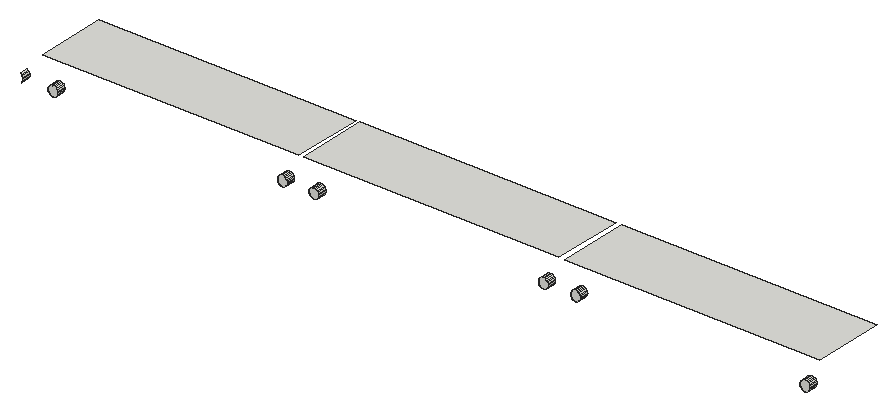
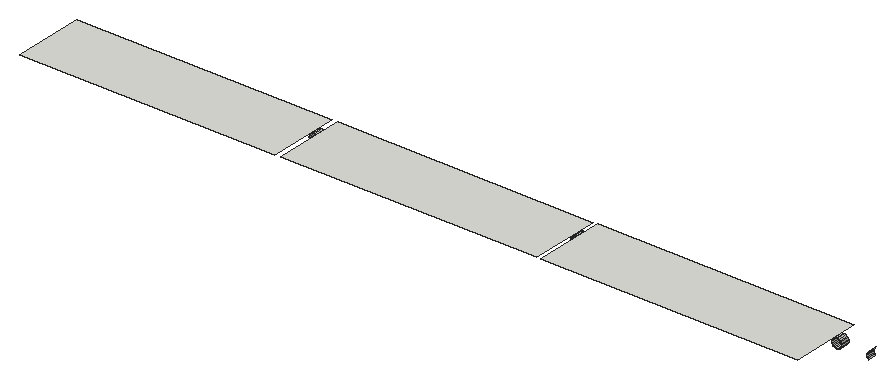
# SketchUp Ruby script. Lengths in inches.
U = 1.inch
M = Sketchup.active_model
def pt(a) = Geom::Point3d.new(a.map { |v| v * U })
def face(e, loops, mat)
  f = e.add_face(loops[0].map { |a| pt(a) })
  loops[1..].each { |l| e.add_face(l.map { |a| pt(a) }).erase! }
  f.material = f.back_material = mat if mat
  f
end
# faces: each face lists its corners as indices into pts; further lists are holes
def faces(e, pts, list, mat = nil) = list.each { |f| face(e, (f[0].is_a?(Array) ? f : [f]).map { |l| l.map { |i| pts[i] } }, mat) }
# xy, xz, yz: faces in a plane at the given z, y or x. An outline is a flat list of corners, or four numbers for a rectangle; further outlines are holes
def ring(l) = l.size == 4 ? [[l[0], l[1]], [l[2], l[1]], [l[2], l[3]], [l[0], l[3]]] : l.each_slice(2).to_a
def flat(e, list, mat, &to3) = list.each { |f| face(e, (f[0].is_a?(Array) ? f : [f]).map { |l| ring(l).map { |u, v| to3.(u, v) } }, mat) }
def xy(e, z, list, mat = nil) = flat(e, list, mat) { |x, y| [x, y, z] }
def xz(e, y, list, mat = nil) = flat(e, list, mat) { |x, z| [x, y, z] }
def yz(e, x, list, mat = nil) = flat(e, list, mat) { |y, z| [x, y, z] }
def lines(e, pts, list) = list.each { |a, b| e.add_line(pt(pts[a]), pt(pts[b])) }
# prism: a flat outline (further loops are holes) pulled along v
def prism(e, loops, v, mat = nil)
  f = face(e, loops, mat); d = Geom::Vector3d.new(v.map { |x| x * U })
  f.pushpull(f.normal.samedirection?(d) ? d.length : -d.length)
end
def box(e, o, s, mat = nil) = prism(e, [[o, [o[0] + s[0], o[1], o[2]], [o[0] + s[0], o[1] + s[1], o[2]], [o[0], o[1] + s[1], o[2]]]], [0, 0, s[2]], mat)
def at(x, y, z, deg = 0) = Geom::Transformation.translation(pt([x, y, z])) * Geom::Transformation.rotation(ORIGIN, Z_AXIS, deg.degrees)
def axes(o, x, y, z) = Geom::Transformation.new([*x, 0, *y, 0, *z, 0, *pt(o).to_a, 1])
def part(name) = M.definitions.add(name)
# library, detail: a bought-in or finely detailed component or shape, given as its bounding box
def library(name, o, s) = part(name).tap { |d| box(d.entities, o, s) }
def detail(e, o, s) = box(e.add_group.entities, o, s)
def put(e, d, t, mat = nil) = e.add_instance(d, t).tap { |i| i.material = mat if mat }
def group(e, t, mat = nil) = e.add_group.tap { |g| g.transformation = t; g.material = mat if mat }.entities
root = M.entities
xy(root,138.0625,[[907.71,801.78,964.82,817.6],[965.89,801.78,1022.875,817.6],[1024.1875,801.78,1080.92,817.6]])
xz(root,799.91,[[911.6,131.88,911.89,131.92,912.16,132.03,912.39,132.21,912.57,132.44,912.68,132.71,912.72,133,912.68,133.29,912.57,133.57,912.39,133.8,912.16,133.98,911.89,134.09,911.6,134.13,911.3,134.09,911.03,133.98,910.8,133.8,910.62,133.57,910.51,133.29,910.47,133,910.51,132.71,910.62,132.44,910.8,132.21,911.03,132.03,911.3,131.92],[962.72,131.88,963.01,131.92,963.28,132.03,963.52,132.21,963.7,132.44,963.81,132.71,963.85,133,963.81,133.29,963.7,133.57,963.52,133.8,963.28,133.98,963.01,134.09,962.72,134.13,962.43,134.09,962.16,133.98,961.93,133.8,961.75,133.57,961.63,133.29,961.6,133,961.63,132.71,961.75,132.44,961.93,132.21,962.16,132.03,962.43,131.92],[969.77,131.88,970.0625,131.92,970.33,132.03,970.57,132.21,970.75,132.44,970.86,132.71,970.9,133,970.86,133.29,970.75,133.57,970.57,133.8,970.33,133.98,970.0625,134.09,969.77,134.13,969.48,134.09,969.21,133.98,968.98,133.8,968.8,133.57,968.69,133.29,968.65,133,968.69,132.71,968.8,132.44,968.98,132.21,969.21,132.03,969.48,131.92],[1020.9,131.88,1021.1875,131.92,1021.46,132.03,1021.69,132.21,1021.87,132.44,1021.98,132.71,1022.02,133,1021.98,133.29,1021.87,133.57,1021.69,133.8,1021.46,133.98,1021.1875,134.09,1020.9,134.13,1020.61,134.09,1020.33,133.98,1020.1,133.8,1019.92,133.57,1019.81,133.29,1019.77,133,1019.81,132.71,1019.92,132.44,1020.1,132.21,1020.33,132.03,1020.61,131.92],[1028.07,131.88,1028.36,131.92,1028.64,132.03,1028.87,132.21,1029.05,132.44,1029.16,132.71,1029.2,133,1029.16,133.29,1029.05,133.57,1028.87,133.8,1028.64,133.98,1028.36,134.09,1028.07,134.13,1027.78,134.09,1027.51,133.98,1027.28,133.8,1027.1,133.57,1026.99,133.29,1026.95,133,1026.99,132.71,1027.1,132.44,1027.28,132.21,1027.51,132.03,1027.78,131.92],
  [1079.2,131.88,1079.49,131.92,1079.76,132.03,1079.99,132.21,1080.17,132.44,1080.28,132.71,1080.32,133,1080.28,133.29,1080.17,133.57,1079.99,133.8,1079.76,133.98,1079.49,134.09,1079.2,134.13,1078.91,134.09,1078.64,133.98,1078.4,133.8,1078.22,133.57,1078.11,133.29,1078.07,133,1078.11,132.71,1078.22,132.44,1078.4,132.21,1078.64,132.03,1078.91,131.92]])
p = [[911.03,801.78,132.03],[911.3,801.78,131.92],[911.3,799.91,131.92],[911.03,799.91,132.03],[911.6,801.78,131.88],[911.6,799.91,131.88],
  [911.89,801.78,131.92],[911.89,799.91,131.92],[912.16,801.78,132.03],[912.16,799.91,132.03],[962.16,801.78,132.03],[962.43,801.78,131.92],
  [962.43,799.91,131.92],[962.16,799.91,132.03],[962.72,801.78,131.88],[962.72,799.91,131.88],[963.01,801.78,131.92],[963.01,799.91,131.92],
  [963.28,801.78,132.03],[963.28,799.91,132.03],[969.21,801.78,132.03],[969.48,801.78,131.92],[969.48,799.91,131.92],[969.21,799.91,132.03],
  [969.77,801.78,131.88],[969.77,799.91,131.88],[970.0625,801.78,131.92],[970.0625,799.91,131.92],[970.33,801.78,132.03],[970.33,799.91,132.03],
  [1020.33,801.78,132.03],[1020.61,801.78,131.92],[1020.61,799.91,131.92],[1020.33,799.91,132.03],[1020.9,801.78,131.88],[1020.9,799.91,131.88],
  [1021.1875,801.78,131.92],[1021.1875,799.91,131.92],[1021.46,801.78,132.03],[1021.46,799.91,132.03],[1027.51,801.78,132.03],[1027.78,801.78,131.92],
  [1027.78,799.91,131.92],[1027.51,799.91,132.03],[1028.07,801.78,131.88],[1028.07,799.91,131.88],[1028.36,801.78,131.92],[1028.36,799.91,131.92],
  [1028.64,801.78,132.03],[1028.64,799.91,132.03],[1078.64,801.78,132.03],[1078.91,801.78,131.92],[1078.91,799.91,131.92],[1078.64,799.91,132.03],
  [1079.2,801.78,131.88],[1079.2,799.91,131.88],[1079.49,801.78,131.92],[1079.49,799.91,131.92],[1079.76,801.78,132.03],[1079.76,799.91,132.03],
  [910.8,801.78,132.21],[910.8,799.91,132.21],[912.39,801.78,132.21],[912.39,799.91,132.21],[961.93,801.78,132.21],[961.93,799.91,132.21],
  [963.52,801.78,132.21],[963.52,799.91,132.21],[968.98,801.78,132.21],[968.98,799.91,132.21],[970.57,801.78,132.21],[970.57,799.91,132.21],
  [1020.1,801.78,132.21],[1020.1,799.91,132.21],[1021.69,801.78,132.21],[1021.69,799.91,132.21],[1027.28,801.78,132.21],[1027.28,799.91,132.21],
  [1028.87,801.78,132.21],[1028.87,799.91,132.21],[1078.4,801.78,132.21],[1078.4,799.91,132.21],[1079.99,801.78,132.21],[1079.99,799.91,132.21],
  [904.53,801.78,132.21],[904.71,801.78,132.44],[904.71,799.91,132.44],[904.53,799.91,132.21],[910.62,801.78,132.44],[910.62,799.91,132.44],
  [912.57,801.78,132.44],[912.57,799.91,132.44],[961.75,801.78,132.44],[961.75,799.91,132.44],[963.7,801.78,132.44],[963.7,799.91,132.44],
  [968.8,801.78,132.44],[968.8,799.91,132.44],[970.75,801.78,132.44],[970.75,799.91,132.44],[1019.92,801.78,132.44],[1019.92,799.91,132.44],
  [1021.87,801.78,132.44],[1021.87,799.91,132.44],[1027.1,801.78,132.44],[1027.1,799.91,132.44],[1029.05,801.78,132.44],[1029.05,799.91,132.44],
  [1078.22,801.78,132.44],[1078.22,799.91,132.44],[1080.17,801.78,132.44],[1080.17,799.91,132.44],[904.82,801.78,132.71],[904.82,799.91,132.71],
  [910.51,801.78,132.71],[910.51,799.91,132.71],[912.68,801.78,132.71],[912.68,799.91,132.71],[961.63,801.78,132.71],[961.63,799.91,132.71],
  [963.81,801.78,132.71],[963.81,799.91,132.71],[968.69,801.78,132.71],[968.69,799.91,132.71],[970.86,801.78,132.71],[970.86,799.91,132.71],
  [1019.81,801.78,132.71],[1019.81,799.91,132.71],[1021.98,801.78,132.71],[1021.98,799.91,132.71],[1026.99,801.78,132.71],[1026.99,799.91,132.71],
  [1029.16,801.78,132.71],[1029.16,799.91,132.71],[1078.11,801.78,132.71],[1078.11,799.91,132.71],[1080.28,801.78,132.71],[1080.28,799.91,132.71],
  [904.86,801.78,133],[904.86,799.91,133],[910.47,801.78,133],[910.47,799.91,133],[912.72,801.78,133],[912.72,799.91,133],
  [961.6,801.78,133],[961.6,799.91,133],[963.85,801.78,133],[963.85,799.91,133],[968.65,801.78,133],[968.65,799.91,133],
  [970.9,801.78,133],[970.9,799.91,133],[1019.77,801.78,133],[1019.77,799.91,133],[1022.02,801.78,133],[1022.02,799.91,133],
  [1026.95,801.78,133],[1026.95,799.91,133],[1029.2,801.78,133],[1029.2,799.91,133],[1078.07,801.78,133],[1078.07,799.91,133],
  [1080.32,801.78,133],[1080.32,799.91,133],[904.82,801.78,133.29],[904.82,799.91,133.29],[910.51,801.78,133.29],[910.51,799.91,133.29],
  [912.68,801.78,133.29],[912.68,799.91,133.29],[961.63,801.78,133.29],[961.63,799.91,133.29],[963.81,801.78,133.29],[963.81,799.91,133.29],
  [968.69,801.78,133.29],[968.69,799.91,133.29],[970.86,801.78,133.29],[970.86,799.91,133.29],[1019.81,801.78,133.29],[1019.81,799.91,133.29],
  [1021.98,801.78,133.29],[1021.98,799.91,133.29],[1026.99,801.78,133.29],[1026.99,799.91,133.29],[1029.16,801.78,133.29],[1029.16,799.91,133.29],
  [1078.11,801.78,133.29],[1078.11,799.91,133.29],[1080.28,801.78,133.29],[1080.28,799.91,133.29],[904.71,801.78,133.57],[904.71,799.91,133.57],
  [910.62,801.78,133.57],[910.62,799.91,133.57],[912.57,801.78,133.57],[912.57,799.91,133.57],[961.75,801.78,133.57],[961.75,799.91,133.57],
  [963.7,801.78,133.57],[963.7,799.91,133.57],[968.8,801.78,133.57],[968.8,799.91,133.57],[970.75,801.78,133.57],[970.75,799.91,133.57],
  [1019.92,801.78,133.57],[1019.92,799.91,133.57],[1021.87,801.78,133.57],[1021.87,799.91,133.57],[1027.1,801.78,133.57],[1027.1,799.91,133.57],
  [1029.05,801.78,133.57],[1029.05,799.91,133.57],[1078.22,801.78,133.57],[1078.22,799.91,133.57],[1080.17,801.78,133.57],[1080.17,799.91,133.57],
  [904.53,801.78,133.8],[904.53,799.91,133.8],[910.8,801.78,133.8],[910.8,799.91,133.8],[912.39,801.78,133.8],[912.39,799.91,133.8],
  [961.93,801.78,133.8],[961.93,799.91,133.8],[963.52,801.78,133.8],[963.52,799.91,133.8],[968.98,801.78,133.8],[968.98,799.91,133.8],
  [970.57,801.78,133.8],[970.57,799.91,133.8],[1020.1,801.78,133.8],[1020.1,799.91,133.8],[1021.69,801.78,133.8],[1021.69,799.91,133.8],
  [1027.28,801.78,133.8],[1027.28,799.91,133.8],[1028.87,801.78,133.8],[1028.87,799.91,133.8],[1078.4,801.78,133.8],[1078.4,799.91,133.8],
  [1079.99,801.78,133.8],[1079.99,799.91,133.8],[904.3,801.78,133.98],[904.3,799.91,133.98],[911.03,801.78,133.98],[911.03,799.91,133.98],
  [912.16,801.78,133.98],[912.16,799.91,133.98],[962.16,801.78,133.98],[962.16,799.91,133.98],[963.28,801.78,133.98],[963.28,799.91,133.98],
  [969.21,801.78,133.98],[969.21,799.91,133.98],[970.33,801.78,133.98],[970.33,799.91,133.98],[1020.33,801.78,133.98],[1020.33,799.91,133.98],
  [1021.46,801.78,133.98],[1021.46,799.91,133.98],[1027.51,801.78,133.98],[1027.51,799.91,133.98],[1028.64,801.78,133.98],[1028.64,799.91,133.98],
  [1078.64,801.78,133.98],[1078.64,799.91,133.98],[1079.76,801.78,133.98],[1079.76,799.91,133.98],[911.3,801.78,134.09],[911.3,799.91,134.09],
  [911.89,801.78,134.09],[911.89,799.91,134.09],[962.43,801.78,134.09],[962.43,799.91,134.09],[963.01,801.78,134.09],[963.01,799.91,134.09],
  [969.48,801.78,134.09],[969.48,799.91,134.09],[970.0625,801.78,134.09],[970.0625,799.91,134.09],[1020.61,801.78,134.09],[1020.61,799.91,134.09],
  [1021.1875,801.78,134.09],[1021.1875,799.91,134.09],[1027.78,801.78,134.09],[1027.78,799.91,134.09],[1028.36,801.78,134.09],[1028.36,799.91,134.09],
  [1078.91,801.78,134.09],[1078.91,799.91,134.09],[1079.49,801.78,134.09],[1079.49,799.91,134.09],[911.6,801.78,134.13],[911.6,799.91,134.13],
  [962.72,801.78,134.13],[962.72,799.91,134.13],[969.77,801.78,134.13],[969.77,799.91,134.13],[1020.9,801.78,134.13],[1020.9,799.91,134.13],
  [1028.07,801.78,134.13],[1028.07,799.91,134.13],[1079.2,801.78,134.13],[1079.2,799.91,134.13]]
faces(root,p,[[0,1,2,3],[1,4,5,2],[4,6,7,5],[6,8,9,7],[10,11,12,13],[11,14,15,12],[14,16,17,15],[16,18,19,17],
  [20,21,22,23],[21,24,25,22],[24,26,27,25],[26,28,29,27],[30,31,32,33],[31,34,35,32],[34,36,37,35],[36,38,39,37],
  [40,41,42,43],[41,44,45,42],[44,46,47,45],[46,48,49,47],[50,51,52,53],[51,54,55,52],[54,56,57,55],[56,58,59,57],
  [60,0,3,61],[8,62,63,9],[64,10,13,65],[18,66,67,19],[68,20,23,69],[28,70,71,29],[72,30,33,73],[38,74,75,39],
  [76,40,43,77],[48,78,79,49],[80,50,53,81],[58,82,83,59],[84,85,86,87],[88,60,61,89],[62,90,91,63],[92,64,65,93],
  [66,94,95,67],[96,68,69,97],[70,98,99,71],[100,72,73,101],[74,102,103,75],[104,76,77,105],[78,106,107,79],[108,80,81,109],
  [82,110,111,83],[85,112,113,86],[114,88,89,115],[90,116,117,91],[118,92,93,119],[94,120,121,95],[122,96,97,123],[98,124,125,99],
  [126,100,101,127],[102,128,129,103],[130,104,105,131],[106,132,133,107],[134,108,109,135],[110,136,137,111],[112,138,139,113],[140,114,115,141],
  [116,142,143,117],[144,118,119,145],[120,146,147,121],[148,122,123,149],[124,150,151,125],[152,126,127,153],[128,154,155,129],[156,130,131,157],
  [132,158,159,133],[160,134,135,161],[136,162,163,137],[138,164,165,139],[166,140,141,167],[142,168,169,143],[170,144,145,171],[146,172,173,147],
  [174,148,149,175],[150,176,177,151],[178,152,153,179],[154,180,181,155],[182,156,157,183],[158,184,185,159],[186,160,161,187],[162,188,189,163],
  [164,190,191,165],[192,166,167,193],[168,194,195,169],[196,170,171,197],[172,198,199,173],[200,174,175,201],[176,202,203,177],[204,178,179,205],
  [180,206,207,181],[208,182,183,209],[184,210,211,185],[212,186,187,213],[188,214,215,189],[190,216,217,191],[218,192,193,219],[194,220,221,195],
  [222,196,197,223],[198,224,225,199],[226,200,201,227],[202,228,229,203],[230,204,205,231],[206,232,233,207],[234,208,209,235],[210,236,237,211],
  [238,212,213,239],[214,240,241,215],[216,242,243,217],[244,218,219,245],[220,246,247,221],[248,222,223,249],[224,250,251,225],[252,226,227,253],
  [228,254,255,229],[256,230,231,257],[232,258,259,233],[260,234,235,261],[236,262,263,237],[264,238,239,265],[240,266,267,241],[268,244,245,269],
  [246,270,271,247],[272,248,249,273],[250,274,275,251],[276,252,253,277],[254,278,279,255],[280,256,257,281],[258,282,283,259],[284,260,261,285],
  [262,286,287,263],[288,264,265,289],[266,290,291,267],[292,268,269,293],[270,292,293,271],[294,272,273,295],[274,294,295,275],[296,276,277,297],
  [278,296,297,279],[298,280,281,299],[282,298,299,283],[300,284,285,301],[286,300,301,287],[302,288,289,303],[290,302,303,291]])
